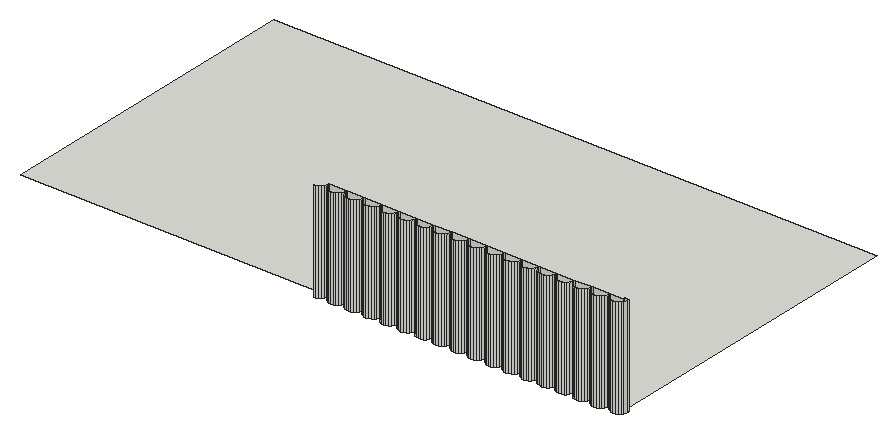
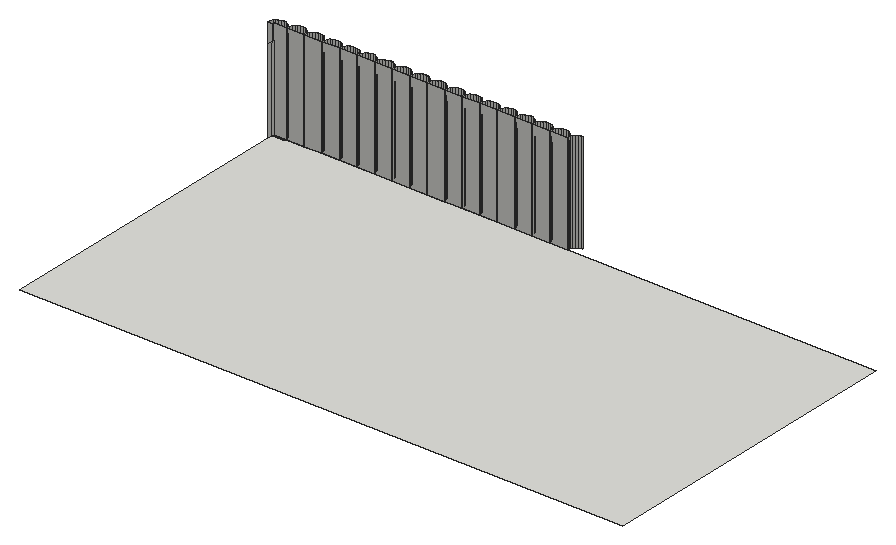
# SketchUp Ruby script. Lengths in inches.
U = 1.inch
M = Sketchup.active_model
def pt(a) = Geom::Point3d.new(a.map { |v| v * U })
def face(e, loops, mat)
  f = e.add_face(loops[0].map { |a| pt(a) })
  loops[1..].each { |l| e.add_face(l.map { |a| pt(a) }).erase! }
  f.material = f.back_material = mat if mat
  f
end
# faces: each face lists its corners as indices into pts; further lists are holes
def faces(e, pts, list, mat = nil) = list.each { |f| face(e, (f[0].is_a?(Array) ? f : [f]).map { |l| l.map { |i| pts[i] } }, mat) }
# xy, xz, yz: faces in a plane at the given z, y or x. An outline is a flat list of corners, or four numbers for a rectangle; further outlines are holes
def ring(l) = l.size == 4 ? [[l[0], l[1]], [l[2], l[1]], [l[2], l[3]], [l[0], l[3]]] : l.each_slice(2).to_a
def flat(e, list, mat, &to3) = list.each { |f| face(e, (f[0].is_a?(Array) ? f : [f]).map { |l| ring(l).map { |u, v| to3.(u, v) } }, mat) }
def xy(e, z, list, mat = nil) = flat(e, list, mat) { |x, y| [x, y, z] }
def xz(e, y, list, mat = nil) = flat(e, list, mat) { |x, z| [x, y, z] }
def yz(e, x, list, mat = nil) = flat(e, list, mat) { |y, z| [x, y, z] }
def lines(e, pts, list) = list.each { |a, b| e.add_line(pt(pts[a]), pt(pts[b])) }
# prism: a flat outline (further loops are holes) pulled along v
def prism(e, loops, v, mat = nil)
  f = face(e, loops, mat); d = Geom::Vector3d.new(v.map { |x| x * U })
  f.pushpull(f.normal.samedirection?(d) ? d.length : -d.length)
end
def box(e, o, s, mat = nil) = prism(e, [[o, [o[0] + s[0], o[1], o[2]], [o[0] + s[0], o[1] + s[1], o[2]], [o[0], o[1] + s[1], o[2]]]], [0, 0, s[2]], mat)
def at(x, y, z, deg = 0) = Geom::Transformation.translation(pt([x, y, z])) * Geom::Transformation.rotation(ORIGIN, Z_AXIS, deg.degrees)
def axes(o, x, y, z) = Geom::Transformation.new([*x, 0, *y, 0, *z, 0, *pt(o).to_a, 1])
def part(name) = M.definitions.add(name)
# library, detail: a bought-in or finely detailed component or shape, given as its bounding box
def library(name, o, s) = part(name).tap { |d| box(d.entities, o, s) }
def detail(e, o, s) = box(e.add_group.entities, o, s)
def put(e, d, t, mat = nil) = e.add_instance(d, t).tap { |i| i.material = mat if mat }
def group(e, t, mat = nil) = e.add_group.tap { |g| g.transformation = t; g.material = mat if mat }.entities
root = M.entities
xy(root,33.18,[[29.4,140.54,29.23,140.5625,29.07,140.63,28.93,140.73,28.83,140.87,28.76,141.03,28.74,141.2,30.05,141.2,30.03,141.03,29.96,140.87,29.86,140.73,29.72,140.63,29.57,140.5625],[30.71,140.54,30.54,140.5625,30.38,140.63,30.24,140.73,30.14,140.87,30.08,141.03,30.05,141.2,31.37,141.2,31.34,141.03,31.28,140.87,31.17,140.73,31.04,140.63,30.88,140.5625],[32.02,140.54,31.85,140.5625,31.69,140.63,31.56,140.73,31.45,140.87,31.39,141.03,31.37,141.2,32.68,141.2,32.66,141.03,32.59,140.87,32.49,140.73,32.35,140.63,32.19,140.5625],[33.33,140.54,33.16,140.5625,33.01,140.63,32.87,140.73,32.77,140.87,32.7,141.03,32.68,141.2,33.99,141.2,33.97,141.03,33.9,140.87,33.8,140.73,33.66,140.63,33.5,140.5625],[34.65,140.54,34.48,140.5625,34.32,140.63,34.18,140.73,34.08,140.87,34.01,141.03,33.99,141.2,35.3,141.2,35.28,141.03,35.21,140.87,35.11,140.73,34.97,140.63,34.82,140.5625],
  [35.96,140.54,35.79,140.5625,35.63,140.63,35.49,140.73,35.39,140.87,35.33,141.03,35.3,141.2,36.62,141.2,36.59,141.03,36.53,140.87,36.42,140.73,36.29,140.63,36.13,140.5625],[37.27,140.54,37.1,140.5625,36.94,140.63,36.81,140.73,36.7,140.87,36.64,141.03,36.62,141.2,37.93,141.2,37.91,141.03,37.84,140.87,37.74,140.73,37.6,140.63,37.44,140.5625],[38.58,140.54,38.41,140.5625,38.26,140.63,38.12,140.73,38.02,140.87,37.95,141.03,37.93,141.2,39.24,141.2,39.22,141.03,39.15,140.87,39.05,140.73,38.91,140.63,38.75,140.5625],[39.9,140.54,39.73,140.5625,39.57,140.63,39.43,140.73,39.33,140.87,39.26,141.03,39.24,141.2,40.55,141.2,40.53,141.03,40.46,140.87,40.36,140.73,40.22,140.63,40.07,140.5625],[41.21,140.54,41.04,140.5625,40.88,140.63,40.74,140.73,40.64,140.87,40.58,141.03,40.55,141.2,41.87,141.2,41.84,141.03,41.78,140.87,41.67,140.73,41.54,140.63,41.38,140.5625],
  [42.52,140.54,42.35,140.5625,42.19,140.63,42.06,140.73,41.95,140.87,41.89,141.03,41.87,141.2,43.18,141.2,43.16,141.03,43.09,140.87,42.99,140.73,42.85,140.63,42.69,140.5625],[43.83,140.54,43.66,140.5625,43.51,140.63,43.37,140.73,43.27,140.87,43.2,141.03,43.18,141.2,44.49,141.2,44.47,141.03,44.4,140.87,44.3,140.73,44.16,140.63,44,140.5625],[45.15,140.54,44.98,140.5625,44.82,140.63,44.68,140.73,44.58,140.87,44.51,141.03,44.49,141.2,45.8,141.2,45.78,141.03,45.71,140.87,45.61,140.73,45.47,140.63,45.32,140.5625],[46.46,140.54,46.29,140.5625,46.13,140.63,45.99,140.73,45.89,140.87,45.83,141.03,45.8,141.2,47.12,141.2,47.09,141.03,47.03,140.87,46.92,140.73,46.79,140.63,46.63,140.5625],[47.77,140.54,47.6,140.5625,47.44,140.63,47.31,140.73,47.2,140.87,47.14,141.03,47.12,141.2,48.43,141.2,48.41,141.03,48.34,140.87,48.24,140.73,48.1,140.63,47.94,140.5625],
  [49.08,140.54,48.91,140.5625,48.76,140.63,48.62,140.73,48.52,140.87,48.45,141.03,48.43,141.2,49.74,141.2,49.72,141.03,49.65,140.87,49.55,140.73,49.41,140.63,49.25,140.5625],[50.375,140.71,50.2,140.73,50.05,140.8,49.91,140.9,49.81,141.04,49.74,141.2,50.74,141.2,50.74,141.37,51.03,141.37,51.01,141.2,50.94,141.04,50.84,140.9,50.7,140.8,50.54,140.73],[5.62,141.2,5.62,164.88,50.74,164.88,50.74,141.37,49.72,141.37,49.74,141.2],[49.74,141.2,49.72,141.37,50.74,141.37,50.74,141.2]])
xz(root,141.2,[[28.74,33.18,30.05,40.6875],[30.05,33.18,31.37,40.6875],[31.37,33.18,32.68,40.6875],[32.68,33.18,33.99,40.6875],[33.99,33.18,35.3,40.6875],
  [35.3,33.18,36.62,40.6875],[36.62,33.18,37.93,40.6875],[37.93,33.18,39.24,40.6875],[39.24,33.18,40.55,40.6875],[40.55,33.18,41.87,40.6875],
  [41.87,33.18,43.18,40.6875],[43.18,33.18,44.49,40.6875],[44.49,33.18,45.8,40.6875],[45.8,33.18,47.12,40.6875],[47.12,33.18,48.43,40.6875],
  [48.43,33.18,49.74,40.6875],[49.74,33.18,50.74,40.6875]])
xz(root,141.37,[[50.74,33.18,51.03,40.6875]])
yz(root,50.74,[[141.2,33.18,141.37,39.45],[141.37,33.18,141.7,39.45]])
p = [[28.08,140.54,33.18],[28.25,140.5625,33.18],[28.25,140.5625,40.6875],[28.08,140.54,40.6875],[29.23,140.5625,33.18],[29.4,140.54,33.18],
  [29.4,140.54,40.6875],[29.23,140.5625,40.6875],[29.57,140.5625,33.18],[29.57,140.5625,40.6875],[30.54,140.5625,33.18],[30.71,140.54,33.18],
  [30.71,140.54,40.6875],[30.54,140.5625,40.6875],[30.88,140.5625,33.18],[30.88,140.5625,40.6875],[31.85,140.5625,33.18],[32.02,140.54,33.18],
  [32.02,140.54,40.6875],[31.85,140.5625,40.6875],[32.19,140.5625,33.18],[32.19,140.5625,40.6875],[33.16,140.5625,33.18],[33.33,140.54,33.18],
  [33.33,140.54,40.6875],[33.16,140.5625,40.6875],[33.5,140.5625,33.18],[33.5,140.5625,40.6875],[34.48,140.5625,33.18],[34.65,140.54,33.18],
  [34.65,140.54,40.6875],[34.48,140.5625,40.6875],[34.82,140.5625,33.18],[34.82,140.5625,40.6875],[35.79,140.5625,33.18],[35.96,140.54,33.18],
  [35.96,140.54,40.6875],[35.79,140.5625,40.6875],[36.13,140.5625,33.18],[36.13,140.5625,40.6875],[37.1,140.5625,33.18],[37.27,140.54,33.18],
  [37.27,140.54,40.6875],[37.1,140.5625,40.6875],[37.44,140.5625,33.18],[37.44,140.5625,40.6875],[38.41,140.5625,33.18],[38.58,140.54,33.18],
  [38.58,140.54,40.6875],[38.41,140.5625,40.6875],[38.75,140.5625,33.18],[38.75,140.5625,40.6875],[39.73,140.5625,33.18],[39.9,140.54,33.18],
  [39.9,140.54,40.6875],[39.73,140.5625,40.6875],[40.07,140.5625,33.18],[40.07,140.5625,40.6875],[41.04,140.5625,33.18],[41.21,140.54,33.18],
  [41.21,140.54,40.6875],[41.04,140.5625,40.6875],[41.38,140.5625,33.18],[41.38,140.5625,40.6875],[42.35,140.5625,33.18],[42.52,140.54,33.18],
  [42.52,140.54,40.6875],[42.35,140.5625,40.6875],[42.69,140.5625,33.18],[42.69,140.5625,40.6875],[43.66,140.5625,33.18],[43.83,140.54,33.18],
  [43.83,140.54,40.6875],[43.66,140.5625,40.6875],[44,140.5625,33.18],[44,140.5625,40.6875],[44.98,140.5625,33.18],[45.15,140.54,33.18],
  [45.15,140.54,40.6875],[44.98,140.5625,40.6875],[45.32,140.5625,33.18],[45.32,140.5625,40.6875],[46.29,140.5625,33.18],[46.46,140.54,33.18],
  [46.46,140.54,40.6875],[46.29,140.5625,40.6875],[46.63,140.5625,33.18],[46.63,140.5625,40.6875],[47.6,140.5625,33.18],[47.77,140.54,33.18],
  [47.77,140.54,40.6875],[47.6,140.5625,40.6875],[47.94,140.5625,33.18],[47.94,140.5625,40.6875],[48.91,140.5625,33.18],[49.08,140.54,33.18],
  [49.08,140.54,40.6875],[48.91,140.5625,40.6875],[49.25,140.5625,33.18],[49.25,140.5625,40.6875],[28.41,140.63,33.18],[28.41,140.63,40.6875],
  [28.55,140.73,33.18],[28.55,140.73,40.6875],[28.93,140.73,33.18],[29.07,140.63,33.18],[29.07,140.63,40.6875],[28.93,140.73,40.6875],
  [29.72,140.63,33.18],[29.72,140.63,40.6875],[29.86,140.73,33.18],[29.86,140.73,40.6875],[30.24,140.73,33.18],[30.38,140.63,33.18],
  [30.38,140.63,40.6875],[30.24,140.73,40.6875],[31.04,140.63,33.18],[31.04,140.63,40.6875],[31.17,140.73,33.18],[31.17,140.73,40.6875],
  [31.56,140.73,33.18],[31.69,140.63,33.18],[31.69,140.63,40.6875],[31.56,140.73,40.6875],[32.35,140.63,33.18],[32.35,140.63,40.6875],
  [32.49,140.73,33.18],[32.49,140.73,40.6875],[32.87,140.73,33.18],[33.01,140.63,33.18],[33.01,140.63,40.6875],[32.87,140.73,40.6875],
  [33.66,140.63,33.18],[33.66,140.63,40.6875],[33.8,140.73,33.18],[33.8,140.73,40.6875],[34.18,140.73,33.18],[34.32,140.63,33.18],
  [34.32,140.63,40.6875],[34.18,140.73,40.6875],[34.97,140.63,33.18],[34.97,140.63,40.6875],[35.11,140.73,33.18],[35.11,140.73,40.6875],
  [35.49,140.73,33.18],[35.63,140.63,33.18],[35.63,140.63,40.6875],[35.49,140.73,40.6875],[36.29,140.63,33.18],[36.29,140.63,40.6875],
  [36.42,140.73,33.18],[36.42,140.73,40.6875],[36.81,140.73,33.18],[36.94,140.63,33.18],[36.94,140.63,40.6875],[36.81,140.73,40.6875],
  [37.6,140.63,33.18],[37.6,140.63,40.6875],[37.74,140.73,33.18],[37.74,140.73,40.6875],[38.12,140.73,33.18],[38.26,140.63,33.18],
  [38.26,140.63,40.6875],[38.12,140.73,40.6875],[38.91,140.63,33.18],[38.91,140.63,40.6875],[39.05,140.73,33.18],[39.05,140.73,40.6875],
  [39.43,140.73,33.18],[39.57,140.63,33.18],[39.57,140.63,40.6875],[39.43,140.73,40.6875],[40.22,140.63,33.18],[40.22,140.63,40.6875],
  [40.36,140.73,33.18],[40.36,140.73,40.6875],[40.74,140.73,33.18],[40.88,140.63,33.18],[40.88,140.63,40.6875],[40.74,140.73,40.6875],
  [41.54,140.63,33.18],[41.54,140.63,40.6875],[41.67,140.73,33.18],[41.67,140.73,40.6875],[42.06,140.73,33.18],[42.19,140.63,33.18],
  [42.19,140.63,40.6875],[42.06,140.73,40.6875],[42.85,140.63,33.18],[42.85,140.63,40.6875],[42.99,140.73,33.18],[42.99,140.73,40.6875],
  [43.37,140.73,33.18],[43.51,140.63,33.18],[43.51,140.63,40.6875],[43.37,140.73,40.6875],[44.16,140.63,33.18],[44.16,140.63,40.6875],
  [44.3,140.73,33.18],[44.3,140.73,40.6875],[44.68,140.73,33.18],[44.82,140.63,33.18],[44.82,140.63,40.6875],[44.68,140.73,40.6875],
  [45.47,140.63,33.18],[45.47,140.63,40.6875],[45.61,140.73,33.18],[45.61,140.73,40.6875],[45.99,140.73,33.18],[46.13,140.63,33.18],
  [46.13,140.63,40.6875],[45.99,140.73,40.6875],[46.79,140.63,33.18],[46.79,140.63,40.6875],[46.92,140.73,33.18],[46.92,140.73,40.6875],
  [47.31,140.73,33.18],[47.44,140.63,33.18],[47.44,140.63,40.6875],[47.31,140.73,40.6875],[48.1,140.63,33.18],[48.1,140.63,40.6875],
  [48.24,140.73,33.18],[48.24,140.73,40.6875],[48.62,140.73,33.18],[48.76,140.63,33.18],[48.76,140.63,40.6875],[48.62,140.73,40.6875],
  [49.41,140.63,33.18],[49.41,140.63,40.6875],[49.55,140.73,33.18],[49.55,140.73,40.6875],[28.65,140.87,33.18],[28.65,140.87,40.6875],
  [28.83,140.87,33.18],[28.83,140.87,40.6875],[29.96,140.87,33.18],[29.96,140.87,40.6875],[30.14,140.87,33.18],[30.14,140.87,40.6875],
  [31.28,140.87,33.18],[31.28,140.87,40.6875],[31.45,140.87,33.18],[31.45,140.87,40.6875],[32.59,140.87,33.18],[32.59,140.87,40.6875],
  [32.77,140.87,33.18],[32.77,140.87,40.6875],[33.9,140.87,33.18],[33.9,140.87,40.6875],[34.08,140.87,33.18],[34.08,140.87,40.6875],
  [35.21,140.87,33.18],[35.21,140.87,40.6875],[35.39,140.87,33.18],[35.39,140.87,40.6875],[36.53,140.87,33.18],[36.53,140.87,40.6875],
  [36.7,140.87,33.18],[36.7,140.87,40.6875],[37.84,140.87,33.18],[37.84,140.87,40.6875],[38.02,140.87,33.18],[38.02,140.87,40.6875],
  [39.15,140.87,33.18],[39.15,140.87,40.6875],[39.33,140.87,33.18],[39.33,140.87,40.6875],[40.46,140.87,33.18],[40.46,140.87,40.6875],
  [40.64,140.87,33.18],[40.64,140.87,40.6875],[41.78,140.87,33.18],[41.78,140.87,40.6875],[41.95,140.87,33.18],[41.95,140.87,40.6875],
  [43.09,140.87,33.18],[43.09,140.87,40.6875],[43.27,140.87,33.18],[43.27,140.87,40.6875],[44.4,140.87,33.18],[44.4,140.87,40.6875],
  [44.58,140.87,33.18],[44.58,140.87,40.6875],[45.71,140.87,33.18],[45.71,140.87,40.6875],[45.89,140.87,33.18],[45.89,140.87,40.6875],
  [47.03,140.87,33.18],[47.03,140.87,40.6875],[47.2,140.87,33.18],[47.2,140.87,40.6875],[48.34,140.87,33.18],[48.34,140.87,40.6875],
  [48.52,140.87,33.18],[48.52,140.87,40.6875],[49.65,140.87,33.18],[49.65,140.87,40.6875],[50.05,140.8,33.18],[50.2,140.73,33.18],
  [50.2,140.73,40.6875],[50.05,140.8,40.6875],[50.375,140.71,33.18],[50.375,140.71,40.6875],[50.54,140.73,33.18],[50.54,140.73,40.6875],
  [50.7,140.8,33.18],[50.7,140.8,40.6875],[49.91,140.9,33.18],[49.91,140.9,40.6875],[50.84,140.9,33.18],[50.84,140.9,40.6875],
  [28.72,141.03,33.18],[28.72,141.03,40.6875],[28.76,141.03,33.18],[28.76,141.03,40.6875],[30.03,141.03,33.18],[30.03,141.03,40.6875],
  [30.08,141.03,33.18],[30.08,141.03,40.6875],[31.34,141.03,33.18],[31.34,141.03,40.6875],[31.39,141.03,33.18],[31.39,141.03,40.6875],
  [32.66,141.03,33.18],[32.66,141.03,40.6875],[32.7,141.03,33.18],[32.7,141.03,40.6875],[33.97,141.03,33.18],[33.97,141.03,40.6875],
  [34.01,141.03,33.18],[34.01,141.03,40.6875],[35.28,141.03,33.18],[35.28,141.03,40.6875],[35.33,141.03,33.18],[35.33,141.03,40.6875],
  [36.59,141.03,33.18],[36.59,141.03,40.6875],[36.64,141.03,33.18],[36.64,141.03,40.6875],[37.91,141.03,33.18],[37.91,141.03,40.6875],
  [37.95,141.03,33.18],[37.95,141.03,40.6875],[39.22,141.03,33.18],[39.22,141.03,40.6875],[39.26,141.03,33.18],[39.26,141.03,40.6875],
  [40.53,141.03,33.18],[40.53,141.03,40.6875],[40.58,141.03,33.18],[40.58,141.03,40.6875],[41.84,141.03,33.18],[41.84,141.03,40.6875],
  [41.89,141.03,33.18],[41.89,141.03,40.6875],[43.16,141.03,33.18],[43.16,141.03,40.6875],[43.2,141.03,33.18],[43.2,141.03,40.6875],
  [44.47,141.03,33.18],[44.47,141.03,40.6875],[44.51,141.03,33.18],[44.51,141.03,40.6875],[45.78,141.03,33.18],[45.78,141.03,40.6875],
  [45.83,141.03,33.18],[45.83,141.03,40.6875],[47.09,141.03,33.18],[47.09,141.03,40.6875],[47.14,141.03,33.18],[47.14,141.03,40.6875],
  [48.41,141.03,33.18],[48.41,141.03,40.6875],[48.45,141.03,33.18],[48.45,141.03,40.6875],[49.72,141.03,33.18],[49.72,141.03,40.6875],
  [49.81,141.04,33.18],[49.81,141.04,40.6875],[50.94,141.04,33.18],[50.94,141.04,40.6875],[28.74,141.2,33.18],[28.74,141.2,40.6875],
  [30.05,141.2,33.18],[30.05,141.2,40.6875],[31.37,141.2,33.18],[31.37,141.2,40.6875],[32.68,141.2,33.18],[32.68,141.2,40.6875],
  [33.99,141.2,33.18],[33.99,141.2,40.6875],[35.3,141.2,33.18],[35.3,141.2,40.6875],[36.62,141.2,33.18],[36.62,141.2,40.6875],
  [37.93,141.2,33.18],[37.93,141.2,40.6875],[39.24,141.2,33.18],[39.24,141.2,40.6875],[40.55,141.2,33.18],[40.55,141.2,40.6875],
  [41.87,141.2,33.18],[41.87,141.2,40.6875],[43.18,141.2,33.18],[43.18,141.2,40.6875],[44.49,141.2,33.18],[44.49,141.2,40.6875],
  [45.8,141.2,33.18],[45.8,141.2,40.6875],[47.12,141.2,33.18],[47.12,141.2,40.6875],[48.43,141.2,33.18],[48.43,141.2,40.6875],
  [49.74,141.2,33.18],[49.74,141.2,40.6875],[51.01,141.2,33.18],[51.01,141.2,39.45],[51.01,141.2,40.6875]]
faces(root,p,[[0,1,2,3],[4,5,6,7],[5,8,9,6],[10,11,12,13],[11,14,15,12],[16,17,18,19],[17,20,21,18],[22,23,24,25],
  [23,26,27,24],[28,29,30,31],[29,32,33,30],[34,35,36,37],[35,38,39,36],[40,41,42,43],[41,44,45,42],[46,47,48,49],
  [47,50,51,48],[52,53,54,55],[53,56,57,54],[58,59,60,61],[59,62,63,60],[64,65,66,67],[65,68,69,66],[70,71,72,73],
  [71,74,75,72],[76,77,78,79],[77,80,81,78],[82,83,84,85],[83,86,87,84],[88,89,90,91],[89,92,93,90],[94,95,96,97],
  [95,98,99,96],[1,100,101,2],[100,102,103,101],[104,105,106,107],[105,4,7,106],[8,108,109,9],[108,110,111,109],[112,113,114,115],
  [113,10,13,114],[14,116,117,15],[116,118,119,117],[120,121,122,123],[121,16,19,122],[20,124,125,21],[124,126,127,125],[128,129,130,131],
  [129,22,25,130],[26,132,133,27],[132,134,135,133],[136,137,138,139],[137,28,31,138],[32,140,141,33],[140,142,143,141],[144,145,146,147],
  [145,34,37,146],[38,148,149,39],[148,150,151,149],[152,153,154,155],[153,40,43,154],[44,156,157,45],[156,158,159,157],[160,161,162,163],
  [161,46,49,162],[50,164,165,51],[164,166,167,165],[168,169,170,171],[169,52,55,170],[56,172,173,57],[172,174,175,173],[176,177,178,179],
  [177,58,61,178],[62,180,181,63],[180,182,183,181],[184,185,186,187],[185,64,67,186],[68,188,189,69],[188,190,191,189],[192,193,194,195],
  [193,70,73,194],[74,196,197,75],[196,198,199,197],[200,201,202,203],[201,76,79,202],[80,204,205,81],[204,206,207,205],[208,209,210,211],
  [209,82,85,210],[86,212,213,87],[212,214,215,213],[216,217,218,219],[217,88,91,218],[92,220,221,93],[220,222,223,221],[224,225,226,227],
  [225,94,97,226],[98,228,229,99],[228,230,231,229],[102,232,233,103],[234,104,107,235],[110,236,237,111],[238,112,115,239],[118,240,241,119],
  [242,120,123,243],[126,244,245,127],[246,128,131,247],[134,248,249,135],[250,136,139,251],[142,252,253,143],[254,144,147,255],[150,256,257,151],
  [258,152,155,259],[158,260,261,159],[262,160,163,263],[166,264,265,167],[266,168,171,267],[174,268,269,175],[270,176,179,271],[182,272,273,183],
  [274,184,187,275],[190,276,277,191],[278,192,195,279],[198,280,281,199],[282,200,203,283],[206,284,285,207],[286,208,211,287],[214,288,289,215],
  [290,216,219,291],[222,292,293,223],[294,224,227,295],[230,296,297,231],[298,299,300,301],[299,302,303,300],[302,304,305,303],[304,306,307,305],
  [308,298,301,309],[306,310,311,307],[232,312,313,233],[314,234,235,315],[236,316,317,237],[318,238,239,319],[240,320,321,241],[322,242,243,323],
  [244,324,325,245],[326,246,247,327],[248,328,329,249],[330,250,251,331],[252,332,333,253],[334,254,255,335],[256,336,337,257],[338,258,259,339],
  [260,340,341,261],[342,262,263,343],[264,344,345,265],[346,266,267,347],[268,348,349,269],[350,270,271,351],[272,352,353,273],[354,274,275,355],
  [276,356,357,277],[358,278,279,359],[280,360,361,281],[362,282,283,363],[284,364,365,285],[366,286,287,367],[288,368,369,289],[370,290,291,371],
  [292,372,373,293],[374,294,295,375],[296,376,377,297],[378,308,309,379],[310,380,381,311],[312,382,383,313],[382,314,315,383],[316,384,385,317],
  [384,318,319,385],[320,386,387,321],[386,322,323,387],[324,388,389,325],[388,326,327,389],[328,390,391,329],[390,330,331,391],[332,392,393,333],
  [392,334,335,393],[336,394,395,337],[394,338,339,395],[340,396,397,341],[396,342,343,397],[344,398,399,345],[398,346,347,399],[348,400,401,349],
  [400,350,351,401],[352,402,403,353],[402,354,355,403],[356,404,405,357],[404,358,359,405],[360,406,407,361],[406,362,363,407],[364,408,409,365],
  [408,366,367,409],[368,410,411,369],[410,370,371,411],[372,412,413,373],[412,374,375,413],[376,414,415,377],[414,378,379,415],[380,416,417,418,381]])
